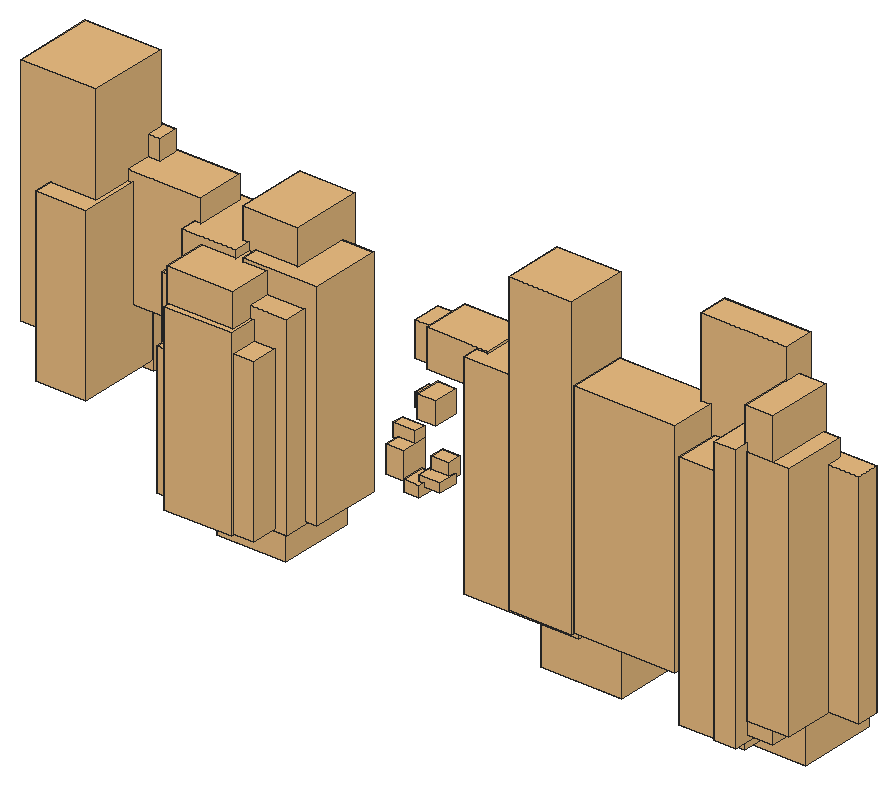
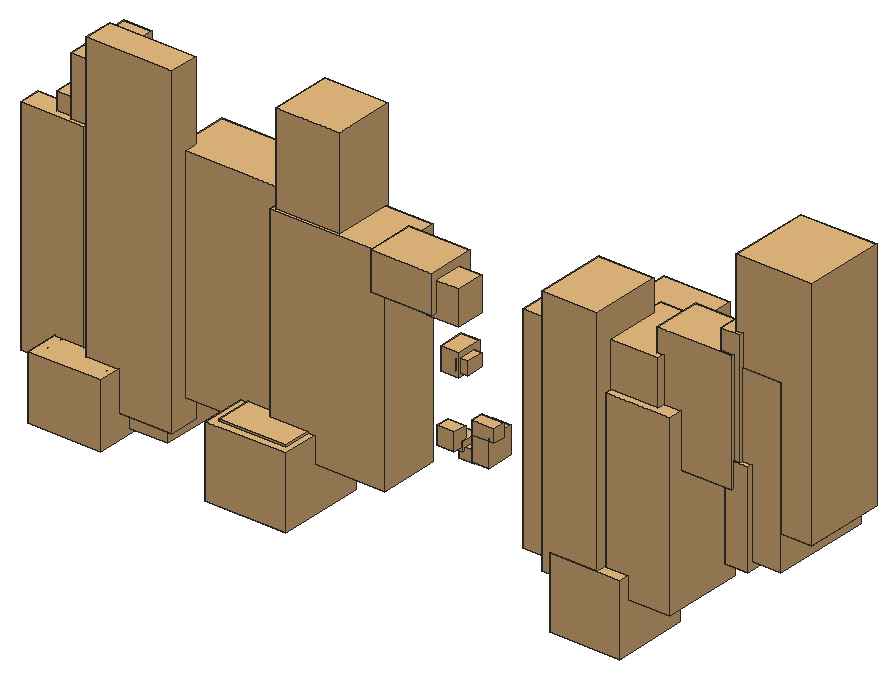
# SketchUp Ruby script. Lengths in inches.
U = 1.inch
M = Sketchup.active_model
def pt(a) = Geom::Point3d.new(a.map { |v| v * U })
def face(e, loops, mat)
  f = e.add_face(loops[0].map { |a| pt(a) })
  loops[1..].each { |l| e.add_face(l.map { |a| pt(a) }).erase! }
  f.material = f.back_material = mat if mat
  f
end
# faces: each face lists its corners as indices into pts; further lists are holes
def faces(e, pts, list, mat = nil) = list.each { |f| face(e, (f[0].is_a?(Array) ? f : [f]).map { |l| l.map { |i| pts[i] } }, mat) }
# xy, xz, yz: faces in a plane at the given z, y or x. An outline is a flat list of corners, or four numbers for a rectangle; further outlines are holes
def ring(l) = l.size == 4 ? [[l[0], l[1]], [l[2], l[1]], [l[2], l[3]], [l[0], l[3]]] : l.each_slice(2).to_a
def flat(e, list, mat, &to3) = list.each { |f| face(e, (f[0].is_a?(Array) ? f : [f]).map { |l| ring(l).map { |u, v| to3.(u, v) } }, mat) }
def xy(e, z, list, mat = nil) = flat(e, list, mat) { |x, y| [x, y, z] }
def xz(e, y, list, mat = nil) = flat(e, list, mat) { |x, z| [x, y, z] }
def yz(e, x, list, mat = nil) = flat(e, list, mat) { |y, z| [x, y, z] }
def lines(e, pts, list) = list.each { |a, b| e.add_line(pt(pts[a]), pt(pts[b])) }
# prism: a flat outline (further loops are holes) pulled along v
def prism(e, loops, v, mat = nil)
  f = face(e, loops, mat); d = Geom::Vector3d.new(v.map { |x| x * U })
  f.pushpull(f.normal.samedirection?(d) ? d.length : -d.length)
end
def box(e, o, s, mat = nil) = prism(e, [[o, [o[0] + s[0], o[1], o[2]], [o[0] + s[0], o[1] + s[1], o[2]], [o[0], o[1] + s[1], o[2]]]], [0, 0, s[2]], mat)
def at(x, y, z, deg = 0) = Geom::Transformation.translation(pt([x, y, z])) * Geom::Transformation.rotation(ORIGIN, Z_AXIS, deg.degrees)
def axes(o, x, y, z) = Geom::Transformation.new([*x, 0, *y, 0, *z, 0, *pt(o).to_a, 1])
def part(name) = M.definitions.add(name)
# library, detail: a bought-in or finely detailed component or shape, given as its bounding box
def library(name, o, s) = part(name).tap { |d| box(d.entities, o, s) }
def detail(e, o, s) = box(e.add_group.entities, o, s)
def put(e, d, t, mat = nil) = e.add_instance(d, t).tap { |i| i.material = mat if mat }
def group(e, t, mat = nil) = e.add_group.tap { |g| g.transformation = t; g.material = mat if mat }.entities
root = M.entities
M.materials.add("BANANA_BIG_STVOL_1").color = [93, 83, 53]
M.materials.add("POT_TEXTURE_1").color = [172, 172, 172]
M.materials.add("soil1").color = [68, 55, 47]
M.materials.add("white_concrete_pot1").color = [212, 211, 204]
c1 = library("Group\#202",[-172.82,-1329.68,294.68],[502.85,397.72,955.79])
c2 = library("Group\#207",[-208.0625,-1498.77,286.27],[547.26,435.76,1075.6])
c3 = library("Group\#203",[-208.33,-1511.76,297.04],[508.2,421.96,1258.76])
c4 = library("Group\#195",[-163.65,-1622.09,292.29],[406.18,374.8,780.12])
c5 = library("Group\#147",[-231.77,1913.24,119.96],[448.93,143.84,1582.05])
c6 = library("Group\#212",[-311.45,-2362.85,663.67],[597.01,322.07,1007.38])
c7 = library("Group\#194",[-208.03,-1336.63,286.21],[381.72,484.79,1145.39])
c8 = library("Group\#149",[-236.03,2064.57,238.29],[378.97,266.89,1422.96])
c9 = library("Group\#145",[-257.06,2048.08,160.05],[394.6,177.93,1743.83])
c10 = library("Group\#220",[-308.37,-2556.11,869.35],[483.58,483.6,1385.8])
c11 = library("Group\#196",[-245.33,-1174.2,301.22],[356.02,306.31,608.34])
c12 = library("Group\#158",[-249.24,914.85,310.18],[345.55,647.95,1307.93])
c13 = library("Group\#142",[-273.21,1593.22,47.51],[374.54,419.07,1416.6])
c14 = library("Group\#155",[-277.97,488.68,287.26],[362.84,405.94,1768.54])
c15 = library("Group\#111",[-143.56,2061.14,371.42],[79.79,63.19,51.3])
c16 = library("Group\#113",[-145.08,2015.32,369.99],[82.29,54.05,37.9])
c17 = library("Group\#106",[-146.29,2044.53,349.125],[81,53.32,37.9])
c18 = library("Group\#92",[-148.5,2084.1,354.63],[73.89,71.73,39.48])
c19 = library("Group\#161",[-299.2,181.55,262.58],[360.65,735.71,1258.34])
c20 = library("Group\#88",[-161.07,2117.49,373.61],[81.25,53.73,39.48])
c21 = library("Group\#133",[-183.79,2161.45,371.25],[72.43,70.21,54.35])
c22 = library("Group\#105",[-200.52,1998.86,370.22],[77.15,68.38,35.39])
c23 = library("Group\#209",[-378.01,-1245.98,305.66],[422.15,474.55,1267.42])
c24 = library("Group\#166",[-249.18,-250.59,980.93],[152.21,116.16,134.05])
c25 = library("Group\#89",[-202.35,1900.5,372.29],[58.53,80.11,50.06])
c26 = library("Group\#204",[-384.8,-1640.99,300.61],[422.68,348.03,1297.96])
c27 = library("Group\#165",[-246.45,-349.05,558.47],[136.91,100.49,66.1])
c28 = library("Group\#183",[-321.08,-139.66,1308.49],[285.55,393.29,221.53])
c29 = library("Group\#199",[-426.76,-1753.59,287.48],[479.67,412.35,1049.19])
c30 = library("Group\#125",[-229.79,1894.04,351.01],[79.82,63.55,37.9])
c31 = library("Group\#172",[-244.55,-305.59,1009.46],[103.13,76.81,77.34])
c32 = library("Group\#134",[-236.3,2186.8,344.47],[79.26,62.91,39.06])
c33 = library("Group\#162",[-258.04,-282.68,604.05],[115.53,137.01,52.63])
c34 = library("Group\#218",[-343.93,-2076.42,1024.91],[285.05,475.82,708.21])
c35 = library("Group\#171",[-292.14,-288.9,1281.79],[169.55,204.34,203.36])
c36 = library("Group\#136",[-234.26,2180.97,367.05],[50.63,74.65,43.95])
c37 = library("Group\#185",[-293.78,-482.77,597.9],[158.75,112.78,159.87])
c38 = library("Group\#151",[-281.17,2118.67,243.77],[133.23,408.71,1313.3])
c39 = library("Group\#115",[-272.7,1884.51,369.99],[80.39,55.87,37.9])
c40 = library("Group\#132",[-275.5,2156.34,352.11],[71.39,73.27,44.69])
c41 = library("Group\#137",[-431.9,1883.46,368.72],[373.65,376.39,18.61])
c42 = library("Group\#117",[-480.58,1843.32,11.96],[467.85,466.24,378.92])
c43 = library("Group\#139",[-312.51,1611.52,263.78],[120.52,408.52,1275.1])
c44 = library("Group\#190",[-429.18,-1441.17,362.05],[345.84,348.28,45.35])
c45 = library("Group\#152",[-468.76,669.89,380.1875],[424.36,427.47,41.99])
c46 = library("Group\#146",[-344.84,1500.61,160.55],[176.35,551.19,1921.45])
c47 = library("Group\#153",[-516.34,626.77,-4.5625],[517.73,515.95,418.98])
c48 = library("Group\#179",[-295.03,-516.52,742.34],[68.71,141.75,78.67])
c49 = library("Group\#191",[-487.23,-1483.58,-4.71],[450.86,446.99,418.38])
c50 = library("Group\#170",[-304.79,-269.16,622.65],[82.06,111.89,102.57])
c51 = library("Group\#208",[-480.32,-1333.42,295.8],[424.49,356.06,1482.77])
c52 = library("Group\#211",[-336.38,-2175.79,614.41],[133.99,147.1,560.64])
c53 = library("Group\#215",[-328.97,-2115.58,1156.29],[117.86,119.42,695.38])
p = [[253.68,273.14,0.11],[253.68,273.11,0.11],[253.7,273.11,0.11]]
lines(root,p,[[0,1],[1,2],[2,0]])
put(root,c1,axes([253.68,273.14,0.11],[0,-0.02318,0],[0.02157,0,0],[0,0,0.02333]))
put(root,c2,axes([253.68,273.14,0.11],[0,-0.02318,0],[0.02157,0,0],[0,0,0.02333]))
put(root,c3,axes([253.68,273.14,0.11],[0,-0.02318,0],[0.02157,0,0],[0,0,0.02333]))
put(root,c4,axes([253.68,273.14,0.11],[0,-0.02318,0],[0.02157,0,0],[0,0,0.02333]))
put(root,c5,axes([253.68,273.14,0.11],[0,-0.02318,0],[0.02157,0,0],[0,0,0.02333]))
put(root,c6,axes([253.68,273.14,0.11],[0,-0.02318,0],[0.02157,0,0],[0,0,0.02333]))
put(root,c7,axes([253.68,273.14,0.11],[0,-0.02318,0],[0.02157,0,0],[0,0,0.02333]))
put(root,c8,axes([253.68,273.14,0.11],[0,-0.02318,0],[0.02157,0,0],[0,0,0.02333]))
put(root,c9,axes([253.68,273.14,0.11],[0,-0.02318,0],[0.02157,0,0],[0,0,0.02333]))
put(root,c10,axes([253.68,273.14,0.11],[0,-0.02318,0],[0.02157,0,0],[0,0,0.02333]))
put(root,c11,axes([253.68,273.14,0.11],[0,-0.02318,0],[0.02157,0,0],[0,0,0.02333]))
put(root,c12,axes([253.68,273.14,0.11],[0,-0.02318,0],[0.02157,0,0],[0,0,0.02333]))
put(root,c13,axes([253.68,273.14,0.11],[0,-0.02318,0],[0.02157,0,0],[0,0,0.02333]))
put(root,c14,axes([253.68,273.14,0.11],[0,-0.02318,0],[0.02157,0,0],[0,0,0.02333]))
g1 = group(root,at(253.68,273.14,0.11),"white_concrete_pot1")
detail(g1,[42.55,1.71,8.4],[1.75,1.29,0.87])
put(root,c15,axes([253.68,273.14,0.11],[0,-0.02318,0],[0.02157,0,0],[0,0,0.02333]),"white_concrete_pot1")
put(root,c16,axes([253.68,273.14,0.11],[0,-0.02318,0],[0.02157,0,0],[0,0,0.02333]),"white_concrete_pot1")
put(root,c17,axes([253.68,273.14,0.11],[0,-0.02318,0],[0.02157,0,0],[0,0,0.02333]),"white_concrete_pot1")
put(root,c18,axes([253.68,273.14,0.11],[0,-0.02318,0],[0.02157,0,0],[0,0,0.02333]),"white_concrete_pot1")
put(root,c19,axes([253.68,273.14,0.11],[0,-0.02318,0],[0.02157,0,0],[0,0,0.02333]))
g2 = group(root,at(253.68,273.14,0.11),"white_concrete_pot1")
detail(g2,[41.78,2.03,8.84],[1.72,1.49,0.87])
put(root,c20,axes([253.68,273.14,0.11],[0,-0.02318,0],[0.02157,0,0],[0,0,0.02333]),"white_concrete_pot1")
g3 = group(root,at(253.68,273.14,0.11),"white_concrete_pot1")
detail(g3,[45.86,2.17,8.27],[1.31,1.86,0.93])
g4 = group(root,at(253.68,273.14,0.11),"white_concrete_pot1")
detail(g4,[41.87,2.35,8.27],[1.67,1.54,0.93])
put(root,c21,axes([253.68,273.14,0.11],[0,-0.02318,0],[0.02157,0,0],[0,0,0.02333]),"white_concrete_pot1")
g5 = group(root,at(253.68,273.14,0.11),"white_concrete_pot1")
detail(g5,[41.27,2.7,7.7],[1.68,1.55,0.92])
put(root,c22,axes([253.68,273.14,0.11],[0,-0.02318,0],[0.02157,0,0],[0,0,0.02333]),"white_concrete_pot1")
g6 = group(root,at(253.68,273.14,0.11),"white_concrete_pot1")
detail(g6,[43.56,3.17,8.66],[1.75,1.37,0.87])
put(root,c23,axes([253.68,273.14,0.11],[0,-0.02318,0],[0.02157,0,0],[0,0,0.02333]))
put(root,c24,axes([253.68,273.14,0.11],[0,-0.02318,0],[0.02157,0,0],[0,0,0.02333]))
put(root,c25,axes([253.68,273.14,0.11],[0,-0.02318,0],[0.02157,0,0],[0,0,0.02333]),"white_concrete_pot1")
put(root,c26,axes([253.68,273.14,0.11],[0,-0.02318,0],[0.02157,0,0],[0,0,0.02333]))
put(root,c27,axes([253.68,273.14,0.11],[0,-0.02318,0],[0.02157,0,0],[0,0,0.02333]))
put(root,c28,axes([253.68,273.14,0.11],[0,-0.02318,0],[0.02157,0,0],[0,0,0.02333]))
g7 = group(root,at(253.68,273.14,0.11),"white_concrete_pot1")
detail(g7,[42.21,3.43,7.7],[1.67,1.55,0.92])
g8 = group(root,at(253.68,273.14,0.11),"white_concrete_pot1")
detail(g8,[42.5,3.68,8.84],[1.75,1.17,0.87])
put(root,c29,axes([253.68,273.14,0.11],[0,-0.02318,0],[0.02157,0,0],[0,0,0.02333]))
put(root,c30,axes([253.68,273.14,0.11],[0,-0.02318,0],[0.02157,0,0],[0,0,0.02333]),"white_concrete_pot1")
g9 = group(root,at(253.68,273.14,0.11),"white_concrete_pot1")
detail(g9,[44.58,3.69,8.4],[1.69,1.48,0.87])
g10 = group(root,at(253.68,273.14,0.11),"white_concrete_pot1")
detail(g10,[45.6875,3.72,8.68],[1.625,1.43,1.18])
put(root,c31,axes([253.68,273.14,0.11],[0,-0.02318,0],[0.02157,0,0],[0,0,0.02333]))
put(root,c32,axes([253.68,273.14,0.11],[0,-0.02318,0],[0.02157,0,0],[0,0,0.02333]),"white_concrete_pot1")
put(root,c33,axes([253.68,273.14,0.11],[0,-0.02318,0],[0.02157,0,0],[0,0,0.02333]))
put(root,c34,axes([253.68,273.14,0.11],[0,-0.02318,0],[0.02157,0,0],[0,0,0.02333]))
g11 = group(root,at(253.68,273.14,0.11),"white_concrete_pot1")
detail(g11,[44.32,3.92,8.84],[1.56,1.66,0.87])
put(root,c35,axes([253.68,273.14,0.11],[0,-0.02318,0],[0.02157,0,0],[0,0,0.02333]))
put(root,c36,axes([253.68,273.14,0.11],[0,-0.02318,0],[0.02157,0,0],[0,0,0.02333]),"white_concrete_pot1")
put(root,c37,axes([253.68,273.14,0.11],[0,-0.02318,0],[0.02157,0,0],[0,0,0.02333]))
put(root,c38,axes([253.68,273.14,0.11],[0,-0.02318,0],[0.02157,0,0],[0,0,0.02333]))
g12 = group(root,at(253.68,273.14,0.11),"white_concrete_pot1")
detail(g12,[45.68,4.45,8.4],[1.75,1.34,0.87])
g13 = group(root,at(253.68,273.14,0.11),"white_concrete_pot1")
detail(g13,[41.49,4.35,8.4],[1.44,1.76,0.87])
put(root,c39,axes([253.68,273.14,0.11],[0,-0.02318,0],[0.02157,0,0],[0,0,0.02333]),"white_concrete_pot1")
put(root,c40,axes([253.68,273.14,0.11],[0,-0.02318,0],[0.02157,0,0],[0,0,0.02333]),"white_concrete_pot1")
g14 = group(root,at(253.68,273.14,0.11),"white_concrete_pot1")
detail(g14,[41.72,4.67,9.09],[1.28,1.88,0.82])
g15 = group(root,at(253.68,273.14,0.11),"white_concrete_pot1")
detail(g15,[41.7,4.73,8.72],[1.19,1.87,0.87])
g16 = group(root,at(253.68,273.14,0.11),"white_concrete_pot1")
detail(g16,[46.95,5.07,8.05],[1.77,1.21,0.9])
put(root,c41,axes([253.68,273.14,0.11],[0,-0.02318,0],[0.02157,0,0],[0,0,0.02333]),"white_concrete_pot1")
put(root,c42,axes([253.68,273.14,0.11],[0,-0.02318,0],[0.02157,0,0],[0,0,0.02333]),"POT_TEXTURE_1")
put(root,c43,axes([253.68,273.14,0.11],[0,-0.02318,0],[0.02157,0,0],[0,0,0.02333]))
put(root,c44,axes([253.68,273.14,0.11],[0,-0.02318,0],[0.02157,0,0],[0,0,0.02333]),"soil1")
put(root,c45,axes([253.68,273.14,0.11],[0,-0.02318,0],[0.02157,0,0],[0,0,0.02333]),"soil1")
put(root,c46,axes([253.68,273.14,0.11],[0,-0.02318,0],[0.02157,0,0],[0,0,0.02333]))
put(root,c47,axes([253.68,273.14,0.11],[0,-0.02318,0],[0.02157,0,0],[0,0,0.02333]),"POT_TEXTURE_1")
put(root,c48,axes([253.68,273.14,0.11],[0,-0.02318,0],[0.02157,0,0],[0,0,0.02333]))
put(root,c49,axes([253.68,273.14,0.11],[0,-0.02318,0],[0.02157,0,0],[0,0,0.02333]),"POT_TEXTURE_1")
put(root,c50,axes([253.68,273.14,0.11],[0,-0.02318,0],[0.02157,0,0],[0,0,0.02333]))
put(root,c51,axes([253.68,273.14,0.11],[0,-0.02318,0],[0.02157,0,0],[0,0,0.02333]))
put(root,c52,axes([253.68,273.14,0.11],[0,-0.02318,0],[0.02157,0,0],[0,0,0.02333]),"BANANA_BIG_STVOL_1")
put(root,c53,axes([253.68,273.14,0.11],[0,-0.02318,0],[0.02157,0,0],[0,0,0.02333]))
